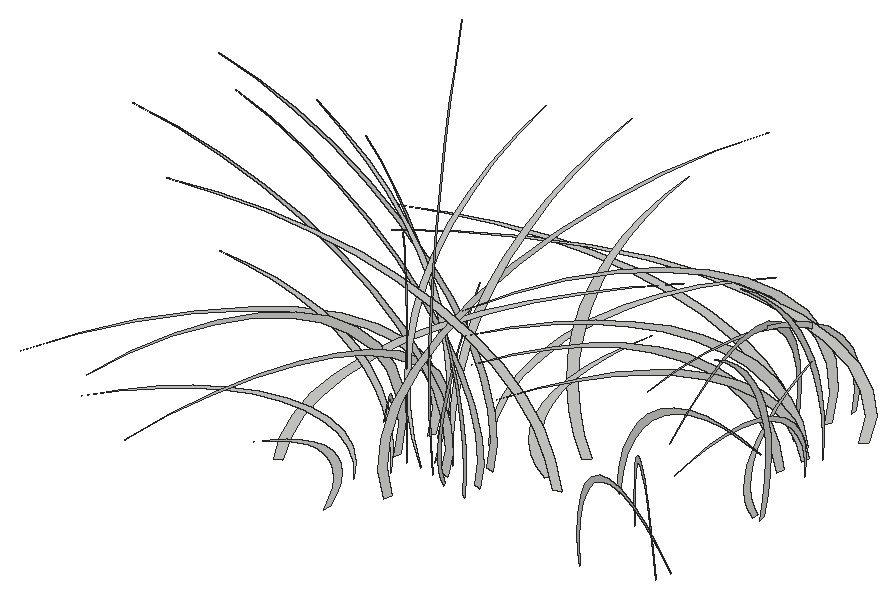
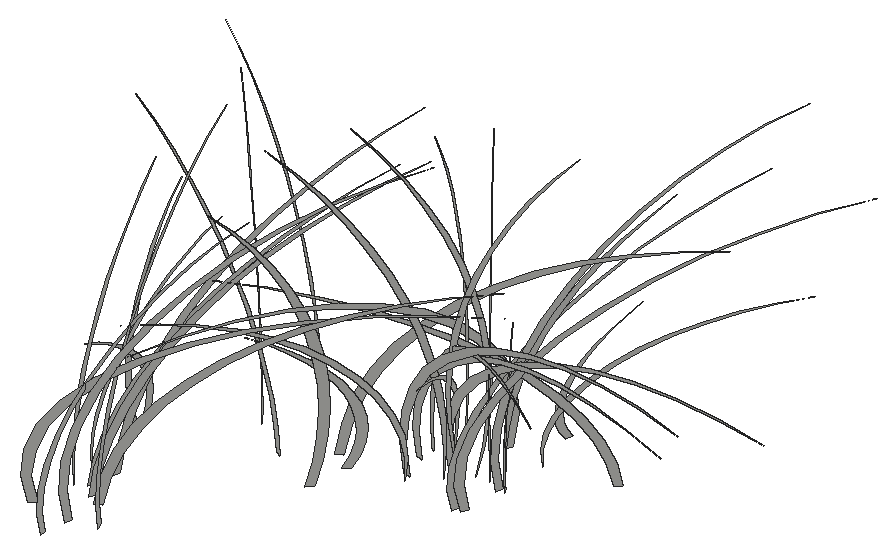
# SketchUp Ruby script. Lengths in inches.
U = 1.inch
M = Sketchup.active_model
def pt(a) = Geom::Point3d.new(a.map { |v| v * U })
def face(e, loops, mat)
  f = e.add_face(loops[0].map { |a| pt(a) })
  loops[1..].each { |l| e.add_face(l.map { |a| pt(a) }).erase! }
  f.material = f.back_material = mat if mat
  f
end
# faces: each face lists its corners as indices into pts; further lists are holes
def faces(e, pts, list, mat = nil) = list.each { |f| face(e, (f[0].is_a?(Array) ? f : [f]).map { |l| l.map { |i| pts[i] } }, mat) }
# xy, xz, yz: faces in a plane at the given z, y or x. An outline is a flat list of corners, or four numbers for a rectangle; further outlines are holes
def ring(l) = l.size == 4 ? [[l[0], l[1]], [l[2], l[1]], [l[2], l[3]], [l[0], l[3]]] : l.each_slice(2).to_a
def flat(e, list, mat, &to3) = list.each { |f| face(e, (f[0].is_a?(Array) ? f : [f]).map { |l| ring(l).map { |u, v| to3.(u, v) } }, mat) }
def xy(e, z, list, mat = nil) = flat(e, list, mat) { |x, y| [x, y, z] }
def xz(e, y, list, mat = nil) = flat(e, list, mat) { |x, z| [x, y, z] }
def yz(e, x, list, mat = nil) = flat(e, list, mat) { |y, z| [x, y, z] }
def lines(e, pts, list) = list.each { |a, b| e.add_line(pt(pts[a]), pt(pts[b])) }
# prism: a flat outline (further loops are holes) pulled along v
def prism(e, loops, v, mat = nil)
  f = face(e, loops, mat); d = Geom::Vector3d.new(v.map { |x| x * U })
  f.pushpull(f.normal.samedirection?(d) ? d.length : -d.length)
end
def box(e, o, s, mat = nil) = prism(e, [[o, [o[0] + s[0], o[1], o[2]], [o[0] + s[0], o[1] + s[1], o[2]], [o[0], o[1] + s[1], o[2]]]], [0, 0, s[2]], mat)
def at(x, y, z, deg = 0) = Geom::Transformation.translation(pt([x, y, z])) * Geom::Transformation.rotation(ORIGIN, Z_AXIS, deg.degrees)
def axes(o, x, y, z) = Geom::Transformation.new([*x, 0, *y, 0, *z, 0, *pt(o).to_a, 1])
def part(name) = M.definitions.add(name)
# library, detail: a bought-in or finely detailed component or shape, given as its bounding box
def library(name, o, s) = part(name).tap { |d| box(d.entities, o, s) }
def detail(e, o, s) = box(e.add_group.entities, o, s)
def put(e, d, t, mat = nil) = e.add_instance(d, t).tap { |i| i.material = mat if mat }
def group(e, t, mat = nil) = e.add_group.tap { |g| g.transformation = t; g.material = mat if mat }.entities
root = M.entities
g1 = group(root,at(15.52,757.05,-58.625))
p = [[-0.0625,-0.5625,0],[-0.03,-0.25,0],[0,0,1.26],[-0.01,-0.1,2.52],[-0.0625,-0.55,3.76],[-0.15,-1.33,4.94],
  [-0.27,-2.43,6.04],[-0.42,-3.83,7.03],[-0.6,-5.47,7.88],[-0.81,-7.33,8.57],[-1.03,-9.36,9.09],[-1.27,-11.51,9.42],
  [-1.51,-13.72,9.56],[-1.76,-15.9375,9.49],[-1.52,-13.76,9.51],[-1.28,-11.6,9.33],[-1.05,-9.52,8.97],[-0.83,-7.55,8.44],
  [-0.63,-5.75,7.74],[-0.46,-4.16,6.89],[-0.31,-2.81,5.92],[-0.19,-1.73,4.84],[-0.11,-0.95,3.68],[-0.05,-0.49,2.47],
  [-0.04,-0.36,1.23]]
faces(g1,p,[[0,1,2,3,4,5,6,7,8,9,10,11,12,13,14,15,16,17,18,19,20,21,22,23,24]])
g2 = group(root,at(15.52,757.05,-58.625))
p = [[-0.0625,-0.5625,0],[-0.03,-0.25,0],[0,0,1.26],[-0.01,-0.1,2.52],[-0.0625,-0.55,3.76],[-0.15,-1.33,4.94],
  [-0.27,-2.43,6.04],[-0.42,-3.83,7.03],[-0.6,-5.47,7.88],[-0.81,-7.33,8.57],[-1.03,-9.36,9.09],[-1.27,-11.51,9.42],
  [-1.51,-13.72,9.56],[-1.76,-15.9375,9.49],[-1.52,-13.76,9.51],[-1.28,-11.6,9.33],[-1.05,-9.52,8.97],[-0.83,-7.55,8.44],
  [-0.63,-5.75,7.74],[-0.46,-4.16,6.89],[-0.31,-2.81,5.92],[-0.19,-1.73,4.84],[-0.11,-0.95,3.68],[-0.05,-0.49,2.47],
  [-0.04,-0.36,1.23]]
faces(g2,p,[[0,1,2,3,4,5,6,7,8,9,10,11,12,13,14,15,16,17,18,19,20,21,22,23,24]])
g3 = group(root,at(15.375,754.41,-58.625))
p = [[-5.63,-8.5625,5.13],[-4.87,-7.41,5.1],[-4.13,-6.28,4.97],[-3.41,-5.1875,4.76],[-2.73,-4.16,4.46],[-2.11,-3.21,4.09],
  [-1.55,-2.36,3.64],[-1.07,-1.62,3.13],[-0.67,-1.02,2.5625],[-0.36,-0.55,1.96],[-0.16,-0.24,1.32],[-0.05,-0.08,0.66],
  [-0.05,-0.08,0],[0,0,0.68],[-0.07,-0.1,1.35],[-0.25,-0.375,2.01],[-0.54,-0.82,2.64],[-0.93,-1.42,3.22],
  [-1.42,-2.16,3.74],[-2,-3.04,4.2],[-2.64,-4.02,4.57],[-3.34,-5.09,4.86],[-4.09,-6.22,5.05],[-4.85,-7.38,5.14]]
faces(g3,p,[[0,1,2,3,4,5,6,7,8,9,10,11,12,13,14,15,16,17,18,19,20,21,22,23]])
g4 = group(root,at(25.16,754.75,-58.625))
p = [[0.39,-0.31,0],[0.18,-0.14,0],[0,0,0.95],[0.07,-0.06,1.9],[0.39,-0.3,2.83],[0.9375,-0.73,3.72],
  [1.71,-1.33,4.55],[2.69,-2.09,5.29],[3.85,-2.99,5.93],[5.16,-4,6.45],[6.58,-5.11,6.84],[8.09,-6.28,7.09],
  [9.65,-7.49,7.1875],[11.21,-8.7,7.14],[9.68,-7.51,7.15],[8.16,-6.33,7.02],[6.69,-5.2,6.75],[5.3125,-4.12,6.35],
  [4.04,-3.14,5.82],[2.92,-2.27,5.18],[1.97,-1.53,4.45],[1.22,-0.94,3.64],[0.67,-0.52,2.77],[0.35,-0.27,1.86],
  [0.25,-0.2,0.93]]
faces(g4,p,[[0,1,2,3,4,5,6,7,8,9,10,11,12,13,14,15,16,17,18,19,20,21,22,23,24]])
g5 = group(root,at(15.86,759.13,-58.625))
p = [[-0.04,-0.6,0],[-0.02,-0.27,0],[0,0,0.91],[-0.01,-0.11,1.82],[-0.04,-0.59,2.72],[-0.09,-1.4375,3.57],
  [-0.16,-2.625,4.37],[-0.25,-4.125,5.08],[-0.35,-5.9,5.69],[-0.47,-7.9,6.19],[-0.6,-10.09,6.57],[-0.74,-12.41,6.81],
  [-0.88,-14.79,6.91],[-1.03,-17.18,6.86],[-0.89,-14.83,6.87],[-0.75,-12.51,6.74],[-0.61,-10.26,6.48],[-0.49,-8.14,6.09],
  [-0.37,-6.2,5.59],[-0.27,-4.48,4.98],[-0.18,-3.03,4.28],[-0.11,-1.87,3.5],[-0.0625,-1.03,2.66],[-0.03,-0.53,1.79],
  [-0.02,-0.39,0.89]]
faces(g5,p,[[0,1,2,3,4,5,6,7,8,9,10,11,12,13,14,15,16,17,18,19,20,21,22,23,24]])
g6 = group(root,at(16.01,752.84,-58.625))
p = [[-0.56,-4.34,4.09],[-0.46,-3.55,3.83],[-0.36,-2.83,3.54],[-0.28,-2.2,3.24],[-0.21,-1.65,2.91],[-0.15,-1.2,2.57],
  [-0.11,-0.85,2.22],[-0.08,-0.6,1.85],[-0.06,-0.45,1.48],[-0.05,-0.41,1.11],[-0.06,-0.47,0.73],[-0.08,-0.64,0.36],
  [-0.12,-0.91,0],[-0.07,-0.56,0],[-0.03,-0.26,0.37],[-0.01,-0.07,0.74],[0,0,1.125],[-0.01,-0.05,1.51],
  [-0.03,-0.21,1.88],[-0.0625,-0.49,2.25],[-0.11,-0.89,2.61],[-0.18,-1.39,2.95],[-0.26,-1.99,3.27],[-0.35,-2.6875,3.57],
  [-0.45,-3.48,3.84]]
faces(g6,p,[[0,1,2,3,4,5,6,7,8,9,10,11,12,13,14,15,16,17,18,19,20,21,22,23,24]])
g7 = group(root,at(15.67,758.97,-58.625))
p = [[-0.23,-0.5625,0],[-0.1,-0.25,0],[0,0,1.07],[-0.04,-0.1,2.14],[-0.22,-0.55,3.2],[-0.54,-1.34,4.2],
  [-0.98,-2.44,5.14],[-1.54,-3.83,5.98],[-2.2,-5.48,6.7],[-2.95,-7.35,7.29],[-3.77,-9.38,7.73],[-4.64,-11.53,8.01],
  [-5.53,-13.75,8.125],[-6.42,-15.97,8.07],[-5.54,-13.79,8.08],[-4.67,-11.625,7.93],[-3.83,-9.54,7.625],[-3.04,-7.57,7.17],
  [-2.32,-5.76,6.58],[-1.67,-4.17,5.86],[-1.13,-2.8125,5.03],[-0.7,-1.73,4.12],[-0.38,-0.96,3.13],[-0.2,-0.49,2.1],
  [-0.15,-0.36,1.05]]
faces(g7,p,[[0,1,2,3,4,5,6,7,8,9,10,11,12,13,14,15,16,17,18,19,20,21,22,23,24]])
g8 = group(root,at(24.9,758.32,-58.625))
p = [[0.36,-0.4,0],[0.16,-0.18,0],[0,0,0.8],[0.0625,-0.07,1.61],[0.35,-0.39,2.4],[0.85,-0.95,3.16],
  [1.54,-1.74,3.86],[2.43,-2.74,4.49],[3.47,-3.91,5.04],[4.65,-5.24,5.48],[5.9375,-6.69,5.8125],[7.3,-8.23,6.02],
  [8.7,-9.81,6.11],[10.11,-11.4,6.07],[8.73,-9.84,6.08],[7.36,-8.3,5.97],[6.04,-6.8,5.74],[4.79,-5.4,5.39],
  [3.65,-4.11,4.95],[2.64,-2.97,4.41],[1.78,-2.01,3.78],[1.1,-1.24,3.1],[0.6,-0.68,2.36],[0.3125,-0.35,1.58],
  [0.23,-0.26,0.79]]
faces(g8,p,[[0,1,2,3,4,5,6,7,8,9,10,11,12,13,14,15,16,17,18,19,20,21,22,23,24]])
g9 = group(root,at(16.14,755.5625,-58.625))
p = [[-3.56,-5.41,10.17],[-2.99,-4.55,9.42],[-2.47,-3.76,8.64],[-2,-3.04,7.84],[-1.57,-2.39,7.02],[-1.2,-1.82,6.18],
  [-0.87,-1.33,5.33],[-0.6,-0.91,4.46],[-0.38,-0.58,3.58],[-0.22,-0.33,2.69],[-0.11,-0.16,1.8],[-0.05,-0.07,0.9],
  [-0.05,-0.07,0],[0,0,0.9],[-0.02,-0.03,1.81],[-0.1,-0.15,2.71],[-0.24,-0.37,3.61],[-0.45,-0.68,4.5],
  [-0.72,-1.09,5.37],[-1.05,-1.59,6.23],[-1.4375,-2.1875,7.07],[-1.88,-2.87,7.89],[-2.39,-3.63,8.68],[-2.95,-4.48,9.4375]]
faces(g9,p,[[0,1,2,3,4,5,6,7,8,9,10,11,12,13,14,15,16,17,18,19,20,21,22,23]])
g10 = group(root,at(15.74,756.88,-58.625))
p = [[0.35,-0.46,0],[0.15,-0.21,1.02],[0.04,-0.05,2.05],[0,0,3.09],[0.04,-0.05,4.12],[0.15,-0.2,5.15],
  [0.34,-0.46,6.17],[0.61,-0.82,7.18],[0.95,-1.27,8.17],[1.36,-1.82,9.14],[1.85,-2.47,10.08],[2.4,-3.21,10.99],
  [3.02,-4.04,11.87],[2.4375,-3.26,10.98],[1.91,-2.5625,10.06],[1.46,-1.95,9.11],[1.0625,-1.42,8.14],[0.73,-0.98,7.16],
  [0.47,-0.63,6.15],[0.28,-0.37,5.14],[0.15,-0.2,4.11],[0.1,-0.13,3.08],[0.11,-0.15,2.05],[0.19,-0.26,1.02]]
faces(g10,p,[[0,1,2,3,4,5,6,7,8,9,10,11,12,13,14,15,16,17,18,19,20,21,22,23]])
g11 = group(root,at(14.75,757.28,-58.625))
p = [[3.37,-4.71,4.09],[2.73,-3.8125,3.83],[2.15,-3,3.54],[1.64,-2.29,3.24],[1.2,-1.67,2.91],[0.83,-1.16,2.57],
  [0.55,-0.77,2.22],[0.35,-0.48,1.85],[0.23,-0.32,1.48],[0.19,-0.27,1.11],[0.24,-0.34,0.73],[0.38,-0.53,0.36],
  [0.6,-0.83,0],[0.45,-0.63,0],[0.2,-0.28,0.36],[0.04,-0.0625,0.73],[-0.02,0.03,1.1],[0.01,-0.01,1.48],
  [0.13,-0.18,1.86],[0.34,-0.48,2.22],[0.65,-0.91,2.58],[1.04,-1.45,2.93],[1.51,-2.11,3.25],[2.0625,-2.88,3.56],
  [2.68,-3.75,3.84]]
faces(g11,p,[[0,1,2,3,4,5,6,7,8,9,10,11,12,13,14,15,16,17,18,19,20,21,22,23,24]])
g12 = group(root,at(21.66,758.23,-58.625))
p = [[-11.7,-4.87,10.21],[-13.47,-5.61,10.48],[-11.76,-4.89,10.15],[-10.11,-4.21,9.7],[-8.53,-3.55,9.13],[-7.05,-2.94,8.44],
  [-5.68,-2.37,7.65],[-4.44,-1.85,6.76],[-3.34,-1.39,5.78],[-2.39,-0.99,4.73],[-1.6,-0.67,3.61],[-0.99,-0.41,2.44],
  [-0.56,-0.23,1.23],[-0.3,-0.125,0],[0,0,0],[-0.21,-0.09,1.26],[-0.61,-0.26,2.5],[-1.22,-0.51,3.7],
  [-2.01,-0.84,4.85],[-2.98,-1.24,5.92],[-4.11,-1.71,6.91],[-5.4,-2.25,7.8],[-6.82,-2.84,8.59],[-8.36,-3.48,9.26],
  [-9.99,-4.16,9.8]]
faces(g12,p,[[0,1,2,3,4,5,6,7,8,9,10,11,12,13,14,15,16,17,18,19,20,21,22,23,24]])
g13 = group(root,at(17.42,757.23,-58.625))
p = [[-0.54,-0.19,0],[-0.24,-0.09,1.2],[-0.0625,-0.02,2.41],[0,0,3.63],[-0.06,-0.02,4.85],[-0.24,-0.09,6.0625],
  [-0.54,-0.19,7.26],[-0.96,-0.34,8.45],[-1.5,-0.53,9.61],[-2.15,-0.76,10.75],[-2.91,-1.03,11.86],[-3.78,-1.34,12.93],
  [-4.75,-1.68,13.96],[-3.84,-1.36,12.92],[-3.01,-1.07,11.83],[-2.29,-0.8125,10.72],[-1.67,-0.59,9.58],[-1.15,-0.41,8.42],
  [-0.74,-0.26,7.24],[-0.4375,-0.15,6.04],[-0.24,-0.09,4.84],[-0.15,-0.05,3.625],[-0.18,-0.0625,2.41],[-0.31,-0.11,1.2]]
faces(g13,p,[[0,1,2,3,4,5,6,7,8,9,10,11,12,13,14,15,16,17,18,19,20,21,22,23]])
g14 = group(root,at(23.11,759.54,-58.625))
p = [[9.9,-5.27,7.86],[11.4,-6.06,8.07],[9.95,-5.29,7.82],[8.55,-4.55,7.47],[7.22,-3.84,7.03],[5.97,-3.17,6.5],
  [4.81,-2.56,5.89],[3.76,-2,5.21],[2.83,-1.5,4.45],[2.02,-1.08,3.64],[1.36,-0.72,2.78],[0.84,-0.45,1.88],
  [0.47,-0.25,0.95],[0.26,-0.14,0],[0,0,0],[0.17,-0.09,0.97],[0.52,-0.28,1.93],[1.03,-0.55,2.85],
  [1.7,-0.9,3.73],[2.52,-1.34,4.56],[3.48,-1.85,5.32],[4.57,-2.43,6.01],[5.77,-3.07,6.61],[7.07,-3.76,7.125],
  [8.46,-4.5,7.54]]
faces(g14,p,[[0,1,2,3,4,5,6,7,8,9,10,11,12,13,14,15,16,17,18,19,20,21,22,23,24]])
g15 = group(root,at(26.84,764.38,-58.625))
p = [[-2.36,-12.45,9.36],[-2.71,-14.33,9.61],[-2.37,-12.51,9.31],[-2.04,-10.75,8.89],[-1.72,-9.08,8.37],[-1.42,-7.5,7.74],
  [-1.15,-6.05,7.02],[-0.89,-4.73,6.2],[-0.67,-3.55,5.3],[-0.48,-2.54,4.34],[-0.32,-1.71,3.3125],[-0.2,-1.05,2.24],
  [-0.11,-0.59,1.13],[-0.0625,-0.32,0],[0,0,0],[-0.04,-0.22,1.16],[-0.125,-0.65,2.3],[-0.25,-1.29,3.39],
  [-0.4,-2.14,4.44],[-0.6,-3.17,5.43],[-0.83,-4.375,6.34],[-1.09,-5.74,7.15],[-1.375,-7.26,7.875],[-1.68,-8.89,8.49],
  [-2.01,-10.63,8.98]]
faces(g15,p,[[0,1,2,3,4,5,6,7,8,9,10,11,12,13,14,15,16,17,18,19,20,21,22,23,24]])
g16 = group(root,at(12.23,753.68,-58.625))
p = [[10.47,7.14,7.55],[12.05,8.22,7.75],[10.52,7.17,7.51],[9.04,6.16,7.17],[7.64,5.2,6.75],[6.3125,4.3,6.24],
  [5.09,3.47,5.66],[3.97,2.71,5],[2.99,2.04,4.28],[2.14,1.46,3.5],[1.44,0.98,2.67],[0.89,0.6,1.81],
  [0.5,0.34,0.91],[0.27,0.1875,0],[0,0,0],[0.18,0.125,0.93],[0.55,0.375,1.85],[1.09,0.74,2.74],
  [1.8,1.22,3.58],[2.66,1.82,4.38],[3.68,2.51,5.11],[4.83,3.29,5.77],[6.1,4.16,6.35],[7.48,5.1,6.85],
  [8.94,6.09,7.25]]
faces(g16,p,[[0,1,2,3,4,5,6,7,8,9,10,11,12,13,14,15,16,17,18,19,20,21,22,23,24]])
g17 = group(root,at(16.3,756.03,-58.625))
p = [[0.41,0.41,0],[0.18,0.18,1.24],[0.05,0.05,2.5],[0,0,3.76],[0.04,0.04,5.02],[0.18,0.18,6.28],
  [0.41,0.41,7.52],[0.72,0.72,8.75],[1.12,1.12,9.96],[1.61,1.61,11.14],[2.18,2.18,12.28],[2.83,2.83,13.39],
  [3.56,3.56,14.46],[2.875,2.875,13.375],[2.26,2.26,12.25],[1.72,1.72,11.1],[1.25,1.25,9.92],[0.87,0.87,8.72],
  [0.56,0.56,7.49],[0.33,0.33,6.26],[0.18,0.18,5.01],[0.12,0.12,3.75],[0.13,0.13,2.5],[0.23,0.23,1.24]]
faces(g17,p,[[0,1,2,3,4,5,6,7,8,9,10,11,12,13,14,15,16,17,18,19,20,21,22,23]])
g18 = group(root,at(18.46,755.22,-58.625))
p = [[-2.35,5.29,5.53],[-1.9,4.29,5.18],[-1.5,3.375,4.79],[-1.14,2.57,4.38],[-0.83,1.88,3.9375],[-0.58,1.31,3.48],
  [-0.38,0.86,3],[-0.24,0.54,2.5],[-0.16,0.36,2],[-0.13,0.3,1.5],[-0.17,0.38,0.99],[-0.26,0.59,0.49],
  [-0.42,0.9375,0],[-0.3125,0.71,0],[-0.14,0.32,0.49],[-0.03,0.07,0.98],[0.02,-0.03,1.49],[0,0.01,2],
  [-0.09,0.2,2.51],[-0.24,0.54,3.01],[-0.45,1.02,3.49],[-0.72,1.63,3.96],[-1.05,2.375,4.4],[-1.4375,3.24,4.81],
  [-1.87,4.22,5.1875]]
faces(g18,p,[[0,1,2,3,4,5,6,7,8,9,10,11,12,13,14,15,16,17,18,19,20,21,22,23,24]])
g19 = group(root,at(18.11,756.48,-58.625))
p = [[-0.6,0.11,0],[-0.26,0.05,0],[0,0,1.07],[-0.11,0.02,2.14],[-0.58,0.1,3.2],[-1.42,0.25,4.2],
  [-2.59,0.46,5.14],[-4.07,0.72,5.98],[-5.82,1.04,6.7],[-7.8,1.39,7.29],[-9.95,1.77,7.73],[-12.23,2.18,8.01],
  [-14.59,2.6,8.125],[-16.95,3.02,8.07],[-14.63,2.61,8.08],[-12.34,2.2,7.93],[-10.12,1.8,7.625],[-8.03,1.43,7.17],
  [-6.12,1.09,6.58],[-4.42,0.79,5.86],[-2.98,0.53,5.03],[-1.84,0.33,4.12],[-1.01,0.18,3.13],[-0.52,0.09,2.1],
  [-0.38,0.07,1.05]]
faces(g19,p,[[0,1,2,3,4,5,6,7,8,9,10,11,12,13,14,15,16,17,18,19,20,21,22,23,24]])
g20 = group(root,at(18.11,756.48,-58.625))
p = [[-0.6,0.11,0],[-0.26,0.05,0],[0,0,1.07],[-0.11,0.02,2.14],[-0.58,0.1,3.2],[-1.42,0.25,4.2],
  [-2.59,0.46,5.14],[-4.07,0.72,5.98],[-5.82,1.04,6.7],[-7.8,1.39,7.29],[-9.95,1.77,7.73],[-12.23,2.18,8.01],
  [-14.59,2.6,8.125],[-16.95,3.02,8.07],[-14.63,2.61,8.08],[-12.34,2.2,7.93],[-10.12,1.8,7.625],[-8.03,1.43,7.17],
  [-6.12,1.09,6.58],[-4.42,0.79,5.86],[-2.98,0.53,5.03],[-1.84,0.33,4.12],[-1.01,0.18,3.13],[-0.52,0.09,2.1],
  [-0.38,0.07,1.05]]
faces(g20,p,[[0,1,2,3,4,5,6,7,8,9,10,11,12,13,14,15,16,17,18,19,20,21,22,23,24]])
g21 = group(root,at(17.57,755.81,-58.625))
p = [[-0.25,0.52,0],[-0.11,0.23,1.38],[-0.03,0.06,2.77],[0,0,4.17],[-0.03,0.06,5.57],[-0.11,0.23,6.97],
  [-0.24,0.52,8.35],[-0.43,0.92,9.71],[-0.67,1.4375,11.05],[-0.97,2.0625,12.36],[-1.31,2.79,13.63],[-1.7,3.63,14.87],
  [-2.14,4.57,16.05],[-1.73,3.68,14.85],[-1.36,2.9,13.6],[-1.03,2.2,12.32],[-0.75,1.61,11.01],[-0.52,1.11,9.68],
  [-0.33,0.71,8.32],[-0.2,0.42,6.94],[-0.11,0.23,5.56],[-0.07,0.15,4.17],[-0.08,0.17,2.77],[-0.14,0.29,1.38]]
faces(g21,p,[[0,1,2,3,4,5,6,7,8,9,10,11,12,13,14,15,16,17,18,19,20,21,22,23]])
g22 = group(root,at(27.06,765.54,-58.625))
p = [[-2.36,-12.45,7.55],[-2.71,-14.33,7.75],[-2.37,-12.51,7.51],[-2.04,-10.75,7.17],[-1.72,-9.08,6.75],[-1.42,-7.5,6.24],
  [-1.15,-6.05,5.66],[-0.89,-4.73,5],[-0.67,-3.55,4.28],[-0.48,-2.54,3.5],[-0.32,-1.71,2.67],[-0.2,-1.05,1.81],
  [-0.11,-0.59,0.91],[-0.0625,-0.32,0],[0,0,0],[-0.04,-0.22,0.93],[-0.125,-0.65,1.85],[-0.25,-1.29,2.74],
  [-0.4,-2.14,3.58],[-0.6,-3.17,4.38],[-0.83,-4.375,5.11],[-1.09,-5.74,5.77],[-1.375,-7.26,6.35],[-1.68,-8.89,6.85],
  [-2.01,-10.63,7.25]]
faces(g22,p,[[0,1,2,3,4,5,6,7,8,9,10,11,12,13,14,15,16,17,18,19,20,21,22,23,24]])
g23 = group(root,at(26.53,766.13,-58.625))
p = [[-3.83,-12.08,8.88],[-4.41,-13.9,9.11],[-3.85,-12.14,8.83],[-3.31,-10.43,8.4375],[-2.79,-8.81,7.94],[-2.31,-7.28,7.34],
  [-1.86,-5.87,6.66],[-1.45,-4.58,5.88],[-1.09,-3.45,5.03],[-0.78,-2.47,4.12],[-0.53,-1.66,3.14],[-0.32,-1.02,2.125],
  [-0.18,-0.57,1.07],[-0.1,-0.31,0],[0,0,0],[-0.07,-0.21,1.1],[-0.2,-0.63,2.18],[-0.4,-1.26,3.22],
  [-0.66,-2.07,4.22],[-0.97,-3.07,5.15],[-1.35,-4.24,6.01],[-1.77,-5.57,6.79],[-2.23,-7.04,7.47],[-2.74,-8.625,8.05],
  [-3.27,-10.3125,8.52]]
faces(g23,p,[[0,1,2,3,4,5,6,7,8,9,10,11,12,13,14,15,16,17,18,19,20,21,22,23,24]])
g24 = group(root,at(19.4375,755.6,-58.625))
p = [[-0.375,0.27,0],[-0.17,0.12,0],[0,0,1.03],[-0.07,0.05,2.06],[-0.37,0.26,3.07],[-0.89,0.64,4.03],
  [-1.63,1.17,4.93],[-2.5625,1.84,5.74],[-3.67,2.63,6.43],[-4.91,3.53,7],[-6.27,4.51,7.42],[-7.71,5.54,7.6875],
  [-9.19,6.6,7.8],[-10.68,7.67,7.75],[-9.22,6.625,7.76],[-7.77,5.59,7.61],[-6.375,4.58,7.32],[-5.06,3.64,6.88],
  [-3.85,2.77,6.3125],[-2.79,2,5.625],[-1.88,1.35,4.83],[-1.16,0.83,3.95],[-0.64,0.46,3.01],[-0.33,0.24,2.02],
  [-0.24,0.17,1.01]]
faces(g24,p,[[0,1,2,3,4,5,6,7,8,9,10,11,12,13,14,15,16,17,18,19,20,21,22,23,24]])
g25 = group(root,at(17.45,757.18,-58.625))
p = [[4.58,4.58,13.75],[3.85,3.85,12.74],[3.18,3.18,11.6875],[2.57,2.57,10.61],[2.02,2.02,9.5],[1.54,1.54,8.36],
  [1.125,1.125,7.21],[0.77,0.77,6.03],[0.49,0.49,4.84],[0.28,0.28,3.64],[0.14,0.14,2.43],[0.0625,0.0625,1.22],
  [0.06,0.06,0],[0,0,1.22],[0.02,0.02,2.45],[0.125,0.125,3.67],[0.3125,0.3125,4.88],[0.58,0.58,6.08],
  [0.92,0.92,7.26],[1.35,1.35,8.42],[1.85,1.85,9.56],[2.43,2.43,10.66],[3.07,3.07,11.73],[3.79,3.79,12.76]]
faces(g25,p,[[0,1,2,3,4,5,6,7,8,9,10,11,12,13,14,15,16,17,18,19,20,21,22,23]])
g26 = group(root,at(19.54,756.45,-58.625))
p = [[-0.57,0.21,0],[-0.25,0.1,0],[0,0,1.07],[-0.1,0.04,2.14],[-0.55,0.21,3.2],[-1.35,0.51,4.2],
  [-2.46,0.93,5.14],[-3.87,1.46,5.98],[-5.53,2.09,6.7],[-7.41,2.8,7.29],[-9.46,3.57,7.73],[-11.625,4.39,8.01],
  [-13.86,5.24,8.125],[-16.1,6.08,8.07],[-13.9,5.25,8.08],[-11.72,4.43,7.93],[-9.62,3.63,7.625],[-7.63,2.88,7.17],
  [-5.81,2.2,6.58],[-4.2,1.59,5.86],[-2.84,1.07,5.03],[-1.75,0.66,4.12],[-0.96,0.36,3.13],[-0.5,0.1875,2.1],
  [-0.37,0.14,1.05]]
faces(g26,p,[[0,1,2,3,4,5,6,7,8,9,10,11,12,13,14,15,16,17,18,19,20,21,22,23,24]])
g27 = group(root,at(27.75,764.53,-58.625))
p = [[2.07,-10.03,5.13],[1.8,-8.68,5.1],[1.52,-7.36,4.97],[1.26,-6.08,4.76],[1.01,-4.87,4.46],[0.78,-3.76,4.09],
  [0.57,-2.76,3.64],[0.39,-1.9,3.13],[0.25,-1.19,2.5625],[0.13,-0.65,1.96],[0.06,-0.28,1.32],[0.02,-0.09,0.66],
  [0.02,-0.09,0],[0,0,0.68],[0.02,-0.12,1.35],[0.09,-0.44,2.01],[0.2,-0.96,2.64],[0.34,-1.66,3.22],
  [0.52,-2.54,3.74],[0.74,-3.56,4.2],[0.97,-4.71,4.57],[1.23,-5.96,4.86],[1.51,-7.29,5.05],[1.79,-8.65,5.14]]
faces(g27,p,[[0,1,2,3,4,5,6,7,8,9,10,11,12,13,14,15,16,17,18,19,20,21,22,23]])
g28 = group(root,at(28.31,761.83,-58.625))
p = [[0.89,-4.29,8.31],[0.72,-3.5,7.78],[0.58,-2.8,7.2],[0.45,-2.17,6.58],[0.34,-1.63,5.92],[0.25,-1.1875,5.22],
  [0.17,-0.84,4.5],[0.12,-0.59,3.76],[0.09,-0.44,3.01],[0.08,-0.4,2.25],[0.1,-0.46,1.49],[0.13,-0.63,0.74],
  [0.19,-0.9,0],[0.11,-0.55,0],[0.05,-0.25,0.75],[0.01,-0.07,1.51],[0,0,2.29],[0.01,-0.05,3.0625],
  [0.04,-0.21,3.83],[0.1,-0.49,4.58],[0.18,-0.875,5.31],[0.28,-1.37,6],[0.41,-1.96,6.65],[0.55,-2.65,7.26],
  [0.71,-3.43,7.82]]
faces(g28,p,[[0,1,2,3,4,5,6,7,8,9,10,11,12,13,14,15,16,17,18,19,20,21,22,23,24]])
g29 = group(root,at(20.17,758.23,-58.625))
p = [[3.1,3.1,5.53],[2.53,2.53,5.18],[2.02,2.02,4.79],[1.57,1.57,4.38],[1.18,1.18,3.9375],[0.86,0.86,3.48],
  [0.61,0.61,3],[0.43,0.43,2.5],[0.32,0.32,2],[0.29,0.29,1.5],[0.34,0.34,0.99],[0.45,0.45,0.49],
  [0.65,0.65,0],[0.4,0.4,0],[0.18,0.18,0.5],[0.05,0.05,1.01],[0,0,1.52],[0.03,0.03,2.04],
  [0.15,0.15,2.55],[0.35,0.35,3.05],[0.63,0.63,3.53],[0.99,0.99,3.99],[1.42,1.42,4.43],[1.92,1.92,4.83],
  [2.48,2.48,5.2]]
faces(g29,p,[[0,1,2,3,4,5,6,7,8,9,10,11,12,13,14,15,16,17,18,19,20,21,22,23,24]])
g30 = group(root,at(24.73,767.97,-58.625))
p = [[0.24,-0.56,0],[0.11,-0.25,0],[0,0,1.07],[0.04,-0.1,2.14],[0.23,-0.55,3.2],[0.57,-1.32,4.2],
  [1.03,-2.42,5.14],[1.62,-3.8,5.98],[2.32,-5.4375,6.7],[3.11,-7.28,7.29],[3.97,-9.3,7.73],[4.875,-11.43,8.01],
  [5.8125,-13.63,8.125],[6.75,-15.83,8.07],[5.83,-13.67,8.08],[4.92,-11.53,7.93],[4.03,-9.45,7.625],[3.2,-7.5,7.17],
  [2.4375,-5.71,6.58],[1.76,-4.13,5.86],[1.1875,-2.79,5.03],[0.73,-1.72,4.12],[0.4,-0.95,3.13],[0.21,-0.49,2.1],
  [0.15,-0.36,1.05]]
faces(g30,p,[[0,1,2,3,4,5,6,7,8,9,10,11,12,13,14,15,16,17,18,19,20,21,22,23,24]])
g31 = group(root,at(19.13,757.72,-58.625))
p = [[-0.58,0.17,0],[-0.26,0.08,0],[0,0,1.23],[-0.1,0.03,2.46],[-0.57,0.17,3.67],[-1.38,0.4,4.83],
  [-2.52,0.74,5.9],[-3.97,1.16,6.87],[-5.67,1.66,7.7],[-7.6,2.22,8.375],[-9.7,2.84,8.88],[-11.93,3.49,9.21],
  [-14.22,4.16,9.34],[-16.52,4.83,9.27],[-14.26,4.17,9.29],[-12.03,3.52,9.12],[-9.87,2.88,8.76],[-7.83,2.29,8.24],
  [-5.96,1.74,7.56],[-4.31,1.26,6.73],[-2.91,0.85,5.78],[-1.79,0.52,4.73],[-0.99,0.29,3.6],[-0.51,0.15,2.41],
  [-0.375,0.11,1.21]]
faces(g31,p,[[0,1,2,3,4,5,6,7,8,9,10,11,12,13,14,15,16,17,18,19,20,21,22,23,24]])
g32 = group(root,at(26.14,768.35,-58.625))
p = [[-0.17,-0.54,0],[-0.08,-0.24,0],[0,0,1.26],[-0.03,-0.1,2.52],[-0.17,-0.53,3.76],[-0.41,-1.28,4.94],
  [-0.74,-2.34,6.04],[-1.16,-3.67,7.03],[-1.66,-5.25,7.88],[-2.23,-7.03,8.57],[-2.85,-8.98,9.09],[-3.5,-11.03,9.42],
  [-4.17,-13.15,9.56],[-4.85,-15.28,9.49],[-4.1875,-13.19,9.51],[-3.53,-11.125,9.33],[-2.9,-9.125,8.97],[-2.3,-7.24,8.44],
  [-1.75,-5.52,7.74],[-1.26,-3.99,6.89],[-0.85,-2.69,5.92],[-0.53,-1.66,4.84],[-0.29,-0.91,3.68],[-0.15,-0.47,2.47],
  [-0.11,-0.35,1.23]]
faces(g32,p,[[0,1,2,3,4,5,6,7,8,9,10,11,12,13,14,15,16,17,18,19,20,21,22,23,24]])
g33 = group(root,at(20.38,760.11,-58.625))
p = [[3.1,3.1,11.24],[2.53,2.53,10.52],[2.02,2.02,9.74],[1.57,1.57,8.9],[1.18,1.18,8],[0.86,0.86,7.07],
  [0.61,0.61,6.09],[0.43,0.43,5.09],[0.32,0.32,4.07],[0.29,0.29,3.04],[0.34,0.34,2.01],[0.45,0.45,1],
  [0.65,0.65,0],[0.4,0.4,0],[0.18,0.18,1.01],[0.05,0.05,2.04],[0,0,3.09],[0.03,0.03,4.14],
  [0.15,0.15,5.18],[0.35,0.35,6.19],[0.63,0.63,7.17],[0.99,0.99,8.11],[1.42,1.42,9],[1.92,1.92,9.82],
  [2.48,2.48,10.57]]
faces(g33,p,[[0,1,2,3,4,5,6,7,8,9,10,11,12,13,14,15,16,17,18,19,20,21,22,23,24]])
g34 = group(root,at(18.43,758.16,-58.625))
p = [[7.25,7.25,6.9375],[6.27,6.27,6.89],[5.3125,5.3125,6.73],[4.39,4.39,6.4375],[3.52,3.52,6.04],[2.71,2.71,5.53],
  [1.99,1.99,4.92],[1.37,1.37,4.23],[0.86,0.86,3.47],[0.47,0.47,2.65],[0.2,0.2,1.78],[0.06,0.06,0.9],
  [0.0625,0.0625,0],[0,0,0.91],[0.08,0.08,1.83],[0.32,0.32,2.72],[0.69,0.69,3.57],[1.2,1.2,4.35],
  [1.83,1.83,5.0625],[2.57,2.57,5.68],[3.4,3.4,6.18],[4.3,4.3,6.57],[5.26,5.26,6.83],[6.25,6.25,6.95]]
faces(g34,p,[[0,1,2,3,4,5,6,7,8,9,10,11,12,13,14,15,16,17,18,19,20,21,22,23]])
g35 = group(root,at(17,753.625,-58.625))
p = [[0.16,0.58,0],[0.07,0.26,0],[0,0,1.23],[0.03,0.11,2.46],[0.15,0.57,3.67],[0.375,1.39,4.83],
  [0.69,2.54,5.9],[1.08,3.99,6.87],[1.54,5.71,7.7],[2.0625,7.65,8.375],[2.63,9.76,8.88],[3.24,12,9.21],
  [3.86,14.3,9.34],[4.48,16.62,9.27],[3.87,14.35,9.29],[3.26,12.1,9.12],[2.68,9.92,8.76],[2.125,7.875,8.24],
  [1.62,6,7.56],[1.17,4.33,6.73],[0.79,2.93,5.78],[0.49,1.8,4.73],[0.27,0.99,3.6],[0.14,0.51,2.41],
  [0.1,0.38,1.21]]
faces(g35,p,[[0,1,2,3,4,5,6,7,8,9,10,11,12,13,14,15,16,17,18,19,20,21,22,23,24]])
g36 = group(root,at(26.07,766.42,-58.625))
p = [[-10.39,-7.25,8.88],[-11.96,-8.35,9.11],[-10.44,-7.29,8.83],[-8.98,-6.26,8.4375],[-7.58,-5.29,7.94],[-6.26,-4.37,7.34],
  [-5.05,-3.52,6.66],[-3.94,-2.75,5.88],[-2.97,-2.07,5.03],[-2.12,-1.48,4.12],[-1.42,-0.99,3.14],[-0.88,-0.61,2.125],
  [-0.49,-0.34,1.07],[-0.27,-0.1875,0],[0,0,0],[-0.18,-0.13,1.1],[-0.54,-0.38,2.18],[-1.08,-0.75,3.22],
  [-1.78,-1.24,4.22],[-2.64,-1.84,5.15],[-3.65,-2.55,6.01],[-4.79,-3.34,6.79],[-6.06,-4.23,7.47],[-7.42,-5.18,8.05],
  [-8.875,-6.19,8.52]]
faces(g36,p,[[0,1,2,3,4,5,6,7,8,9,10,11,12,13,14,15,16,17,18,19,20,21,22,23,24]])
g37 = group(root,at(28.16,760.46,-58.625))
yz(g37,0,[[0.5,0,0.23,0.44,0.0625,0.89,0,1.35,0.04,1.8,0.19,2.25,0.44,2.7,0.79,3.125,1.24,3.53,1.78,3.92,2.4,4.27,3.1,4.6,3.875,4.89,3.17,4.58,2.53,4.24,1.96,3.875,1.48,3.48,1.07,3.08,0.76,2.65,0.53,2.22,0.4,1.77,0.36,1.32,0.42,0.875,0.57,0.43,0.8125,0]])
g38 = group(root,at(27.47,765.88,-58.625))
p = [[1.3125,-6.34,10.17],[1.1,-5.33,9.42],[0.91,-4.4,8.64],[0.74,-3.56,7.84],[0.58,-2.8,7.02],[0.44,-2.13,6.18],
  [0.32,-1.56,5.33],[0.22,-1.07,4.46],[0.14,-0.68,3.58],[0.08,-0.39,2.69],[0.04,-0.1875,1.8],[0.02,-0.09,0.9],
  [0.02,-0.08,0],[0,0,0.9],[0.01,-0.03,1.81],[0.04,-0.17,2.71],[0.09,-0.43,3.61],[0.17,-0.8,4.5],
  [0.26,-1.28,5.37],[0.39,-1.87,6.23],[0.53,-2.5625,7.07],[0.69,-3.36,7.89],[0.88,-4.26,8.68],[1.09,-5.25,9.4375]]
faces(g38,p,[[0,1,2,3,4,5,6,7,8,9,10,11,12,13,14,15,16,17,18,19,20,21,22,23]])
g39 = group(root,at(26.17,769.54,-58.625))
p = [[0.03,-0.46,0],[0.01,-0.21,0],[0,0,0.89],[0.01,-0.08,1.79],[0.03,-0.45,2.67],[0.07,-1.1,3.51],
  [0.13,-2,4.29],[0.2,-3.15,4.99],[0.29,-4.5,5.59],[0.39,-6.04,6.09],[0.5,-7.71,6.45],[0.61,-9.47,6.69],
  [0.73,-11.29,6.79],[0.85,-13.12,6.74],[0.73,-11.33,6.75],[0.62,-9.55,6.625],[0.51,-7.84,6.37],[0.4,-6.22,5.99],
  [0.31,-4.73,5.49],[0.22,-3.42,4.89],[0.15,-2.31,4.2],[0.09,-1.42,3.4375],[0.05,-0.78,2.62],[0.03,-0.41,1.75],
  [0.02,-0.3,0.875]]
faces(g39,p,[[0,1,2,3,4,5,6,7,8,9,10,11,12,13,14,15,16,17,18,19,20,21,22,23,24]])
g40 = group(root,at(28.22,767.92,-58.625))
p = [[-0.5,-0.35,0],[-0.22,-0.15,0],[0,0,1.07],[-0.09,-0.0625,2.14],[-0.49,-0.34,3.2],[-1.18,-0.82,4.2],
  [-2.16,-1.5,5.14],[-3.39,-2.36,5.98],[-4.85,-3.38,6.7],[-6.49,-4.53,7.29],[-8.29,-5.78,7.73],[-10.19,-7.11,8.01],
  [-12.15,-8.48,8.125],[-14.12,-9.85,8.07],[-12.1875,-8.5,8.08],[-10.28,-7.17,7.93],[-8.43,-5.88,7.625],[-6.6875,-4.67,7.17],
  [-5.09,-3.55,6.58],[-3.68,-2.57,5.86],[-2.49,-1.73,5.03],[-1.53,-1.07,4.12],[-0.84,-0.59,3.13],[-0.4375,-0.31,2.1],
  [-0.32,-0.22,1.05]]
faces(g40,p,[[0,1,2,3,4,5,6,7,8,9,10,11,12,13,14,15,16,17,18,19,20,21,22,23,24]])
g41 = group(root,at(28.22,767.92,-58.625))
p = [[-0.5,-0.35,0],[-0.22,-0.15,0],[0,0,1.07],[-0.09,-0.0625,2.14],[-0.49,-0.34,3.2],[-1.18,-0.82,4.2],
  [-2.16,-1.5,5.14],[-3.39,-2.36,5.98],[-4.85,-3.38,6.7],[-6.49,-4.53,7.29],[-8.29,-5.78,7.73],[-10.19,-7.11,8.01],
  [-12.15,-8.48,8.125],[-14.12,-9.85,8.07],[-12.1875,-8.5,8.08],[-10.28,-7.17,7.93],[-8.43,-5.88,7.625],[-6.6875,-4.67,7.17],
  [-5.09,-3.55,6.58],[-3.68,-2.57,5.86],[-2.49,-1.73,5.03],[-1.53,-1.07,4.12],[-0.84,-0.59,3.13],[-0.4375,-0.31,2.1],
  [-0.32,-0.22,1.05]]
faces(g41,p,[[0,1,2,3,4,5,6,7,8,9,10,11,12,13,14,15,16,17,18,19,20,21,22,23,24]])
